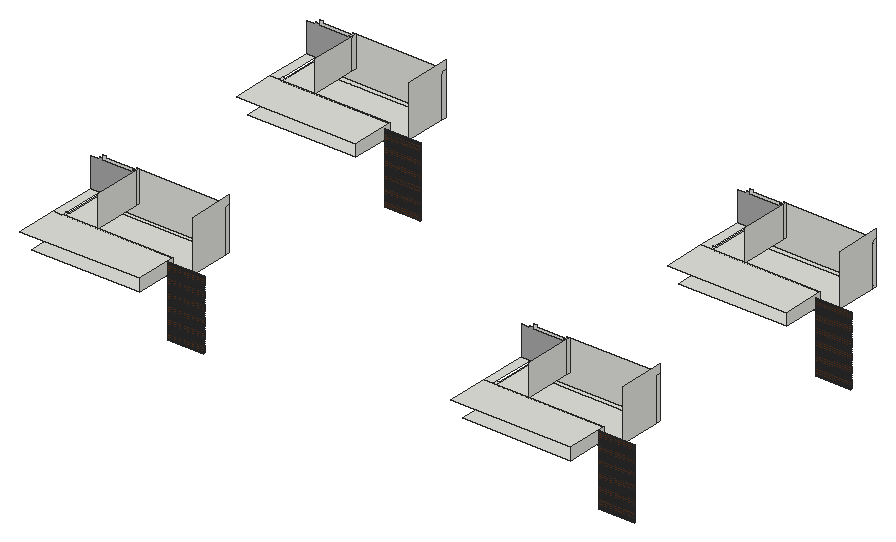
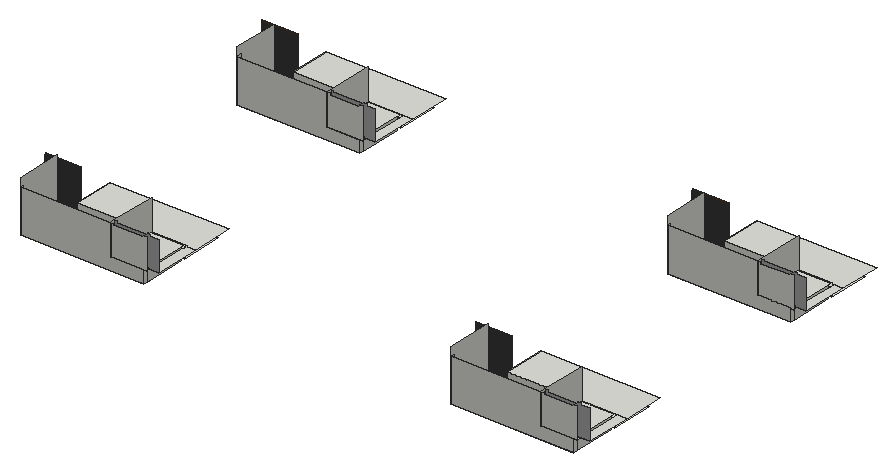
# SketchUp Ruby script. Lengths in inches.
U = 1.inch
M = Sketchup.active_model
def pt(a) = Geom::Point3d.new(a.map { |v| v * U })
def face(e, loops, mat)
  f = e.add_face(loops[0].map { |a| pt(a) })
  loops[1..].each { |l| e.add_face(l.map { |a| pt(a) }).erase! }
  f.material = f.back_material = mat if mat
  f
end
# faces: each face lists its corners as indices into pts; further lists are holes
def faces(e, pts, list, mat = nil) = list.each { |f| face(e, (f[0].is_a?(Array) ? f : [f]).map { |l| l.map { |i| pts[i] } }, mat) }
# xy, xz, yz: faces in a plane at the given z, y or x. An outline is a flat list of corners, or four numbers for a rectangle; further outlines are holes
def ring(l) = l.size == 4 ? [[l[0], l[1]], [l[2], l[1]], [l[2], l[3]], [l[0], l[3]]] : l.each_slice(2).to_a
def flat(e, list, mat, &to3) = list.each { |f| face(e, (f[0].is_a?(Array) ? f : [f]).map { |l| ring(l).map { |u, v| to3.(u, v) } }, mat) }
def xy(e, z, list, mat = nil) = flat(e, list, mat) { |x, y| [x, y, z] }
def xz(e, y, list, mat = nil) = flat(e, list, mat) { |x, z| [x, y, z] }
def yz(e, x, list, mat = nil) = flat(e, list, mat) { |y, z| [x, y, z] }
def lines(e, pts, list) = list.each { |a, b| e.add_line(pt(pts[a]), pt(pts[b])) }
# prism: a flat outline (further loops are holes) pulled along v
def prism(e, loops, v, mat = nil)
  f = face(e, loops, mat); d = Geom::Vector3d.new(v.map { |x| x * U })
  f.pushpull(f.normal.samedirection?(d) ? d.length : -d.length)
end
def box(e, o, s, mat = nil) = prism(e, [[o, [o[0] + s[0], o[1], o[2]], [o[0] + s[0], o[1] + s[1], o[2]], [o[0], o[1] + s[1], o[2]]]], [0, 0, s[2]], mat)
def at(x, y, z, deg = 0) = Geom::Transformation.translation(pt([x, y, z])) * Geom::Transformation.rotation(ORIGIN, Z_AXIS, deg.degrees)
def axes(o, x, y, z) = Geom::Transformation.new([*x, 0, *y, 0, *z, 0, *pt(o).to_a, 1])
def part(name) = M.definitions.add(name)
# library, detail: a bought-in or finely detailed component or shape, given as its bounding box
def library(name, o, s) = part(name).tap { |d| box(d.entities, o, s) }
def detail(e, o, s) = box(e.add_group.entities, o, s)
def put(e, d, t, mat = nil) = e.add_instance(d, t).tap { |i| i.material = mat if mat }
def group(e, t, mat = nil) = e.add_group.tap { |g| g.transformation = t; g.material = mat if mat }.entities
root = M.entities
M.materials.add("[Color M03]1").color = [170, 170, 170]
M.materials.add("[Wood Veneer 01]").color = [96, 56, 29]
c1 = library("A$C06767DEF\#1",[-8.3,1.21,0],[7.09,7.09,5.51])
xy(root,266.84,[[534.24,466.33,620.86,468.64],[1582.55,466.33,1669.17,468.64]])
xy(root,267.22,[[533.89,1125.42,620.51,1127.73],[1582.21,1125.42,1668.82,1127.73]])
xy(root,267.875,[[534.24,466.33,620.86,468.64],[1582.55,466.33,1669.17,468.64]])
xy(root,268.25,[[533.89,1125.42,620.51,1127.73],[1582.21,1125.42,1668.82,1127.73]])
xy(root,270.91,[[534.24,466.33,620.86,468.64],[1582.55,466.33,1669.17,468.64]])
xy(root,271.28,[[533.89,1125.42,620.51,1127.73],[1582.21,1125.42,1668.82,1127.73]])
xy(root,271.9375,[[534.24,466.33,620.86,468.64],[1582.55,466.33,1669.17,468.64]])
xy(root,272.3125,[[533.89,1125.42,620.51,1127.73],[1582.21,1125.42,1668.82,1127.73]])
xy(root,274.97,[[534.24,466.33,620.86,468.64],[1582.55,466.33,1669.17,468.64]])
xy(root,275.34,[[533.89,1125.42,620.51,1127.73],[1582.21,1125.42,1668.82,1127.73]])
xy(root,276,[[534.24,466.33,620.86,468.64],[1582.55,466.33,1669.17,468.64]])
xy(root,276.375,[[533.89,1125.42,620.51,1127.73],[1582.21,1125.42,1668.82,1127.73]])
xy(root,279.03,[[534.24,466.33,620.86,468.64],[1582.55,466.33,1669.17,468.64]])
xy(root,279.41,[[533.89,1125.42,620.51,1127.73],[1582.21,1125.42,1668.82,1127.73]])
xy(root,280.0625,[[534.24,466.33,620.86,468.64],[1582.55,466.33,1669.17,468.64]])
xy(root,280.4375,[[533.89,1125.42,620.51,1127.73],[1582.21,1125.42,1668.82,1127.73]])
xy(root,283.09,[[534.24,466.33,620.86,468.64],[1582.55,466.33,1669.17,468.64]])
xy(root,283.47,[[533.89,1125.42,620.51,1127.73],[1582.21,1125.42,1668.82,1127.73]])
xy(root,284.125,[[534.24,466.33,620.86,468.64],[1582.55,466.33,1669.17,468.64]])
xy(root,284.5,[[533.89,1125.42,620.51,1127.73],[1582.21,1125.42,1668.82,1127.73]])
xy(root,287.16,[[534.24,466.33,620.86,468.64],[1582.55,466.33,1669.17,468.64]])
xy(root,287.53,[[533.89,1125.42,620.51,1127.73],[1582.21,1125.42,1668.82,1127.73]])
xy(root,288.1875,[[534.24,466.33,620.86,468.64],[1582.55,466.33,1669.17,468.64]])
xy(root,288.5625,[[533.89,1125.42,620.51,1127.73],[1582.21,1125.42,1668.82,1127.73]])
xy(root,291.22,[[534.24,466.33,620.86,468.64],[1582.55,466.33,1669.17,468.64]])
xy(root,291.59,[[533.89,1125.42,620.51,1127.73],[1582.21,1125.42,1668.82,1127.73]])
xy(root,292.25,[[534.24,466.33,620.86,468.64],[1582.55,466.33,1669.17,468.64]])
xy(root,292.625,[[533.89,1125.42,620.51,1127.73],[1582.21,1125.42,1668.82,1127.73]])
xy(root,295.28,[[534.24,466.33,620.86,468.64],[1582.55,466.33,1669.17,468.64]])
xy(root,295.66,[[533.89,1125.42,620.51,1127.73],[1582.21,1125.42,1668.82,1127.73]])
xy(root,296.3125,[[534.24,466.33,620.86,468.64],[1582.55,466.33,1669.17,468.64]])
xy(root,296.6875,[[533.89,1125.42,620.51,1127.73],[1582.21,1125.42,1668.82,1127.73]])
xy(root,299.34,[[534.24,466.33,620.86,468.64],[1582.55,466.33,1669.17,468.64]])
xy(root,299.72,[[533.89,1125.42,620.51,1127.73],[1582.21,1125.42,1668.82,1127.73]])
xy(root,300.375,[[534.24,466.33,620.86,468.64],[1582.55,466.33,1669.17,468.64]])
xy(root,300.75,[[533.89,1125.42,620.51,1127.73],[1582.21,1125.42,1668.82,1127.73]])
xy(root,303.41,[[534.24,466.33,620.86,468.64],[1582.55,466.33,1669.17,468.64]])
xy(root,303.78,[[533.89,1125.42,620.51,1127.73],[1582.21,1125.42,1668.82,1127.73]])
xy(root,304.4375,[[534.24,466.33,620.86,468.64],[1582.55,466.33,1669.17,468.64]])
xy(root,304.8125,[[533.89,1125.42,620.51,1127.73],[1582.21,1125.42,1668.82,1127.73]])
xy(root,307.47,[[534.24,466.33,620.86,468.64],[1582.55,466.33,1669.17,468.64]])
xy(root,307.84,[[533.89,1125.42,620.51,1127.73],[1582.21,1125.42,1668.82,1127.73]])
xy(root,308.5,[[534.24,466.33,620.86,468.64],[1582.55,466.33,1669.17,468.64]])
xy(root,308.875,[[533.89,1125.42,620.51,1127.73],[1582.21,1125.42,1668.82,1127.73]])
xy(root,311.53,[[534.24,466.33,620.86,468.64],[1582.55,466.33,1669.17,468.64]])
xy(root,311.91,[[533.89,1125.42,620.51,1127.73],[1582.21,1125.42,1668.82,1127.73]])
xy(root,312.5625,[[534.24,466.33,620.86,468.64],[1582.55,466.33,1669.17,468.64]])
xy(root,312.9375,[[533.89,1125.42,620.51,1127.73],[1582.21,1125.42,1668.82,1127.73]])
xy(root,315.59,[[534.24,466.33,620.86,468.64],[1582.55,466.33,1669.17,468.64]])
xy(root,315.97,[[533.89,1125.42,620.51,1127.73],[1582.21,1125.42,1668.82,1127.73]])
xy(root,316.625,[[534.24,466.33,620.86,468.64],[1582.55,466.33,1669.17,468.64]])
xy(root,317,[[533.89,1125.42,620.51,1127.73],[1582.21,1125.42,1668.82,1127.73]])
xy(root,319.66,[[534.24,466.33,620.86,468.64],[1582.55,466.33,1669.17,468.64]])
xy(root,320.03,[[533.89,1125.42,620.51,1127.73],[1582.21,1125.42,1668.82,1127.73]])
xy(root,320.6875,[[534.24,466.33,620.86,468.64],[1582.55,466.33,1669.17,468.64]])
xy(root,321.0625,[[533.89,1125.42,620.51,1127.73],[1582.21,1125.42,1668.82,1127.73]])
xy(root,323.72,[[534.24,466.33,620.86,468.64],[1582.55,466.33,1669.17,468.64]])
xy(root,324.09,[[533.89,1125.42,620.51,1127.73],[1582.21,1125.42,1668.82,1127.73]])
xy(root,324.75,[[534.24,466.33,620.86,468.64],[1582.55,466.33,1669.17,468.64]])
xy(root,325.125,[[533.89,1125.42,620.51,1127.73],[1582.21,1125.42,1668.82,1127.73]])
xy(root,327.78,[[534.24,466.33,620.86,468.64],[1582.55,466.33,1669.17,468.64]])
xy(root,328.16,[[533.89,1125.42,620.51,1127.73],[1582.21,1125.42,1668.82,1127.73]])
xy(root,328.8125,[[534.24,466.33,620.86,468.64],[1582.55,466.33,1669.17,468.64]])
xy(root,329.1875,[[533.89,1125.42,620.51,1127.73],[1582.21,1125.42,1668.82,1127.73]])
xy(root,331.84,[[534.24,466.33,620.86,468.64],[1582.55,466.33,1669.17,468.64]])
xy(root,332.22,[[533.89,1125.42,620.51,1127.73],[1582.21,1125.42,1668.82,1127.73]])
xy(root,332.875,[[534.24,466.33,620.86,468.64],[1582.55,466.33,1669.17,468.64]])
xy(root,333.25,[[533.89,1125.42,620.51,1127.73],[1582.21,1125.42,1668.82,1127.73]])
xy(root,335.91,[[534.24,466.33,620.86,468.64],[1582.55,466.33,1669.17,468.64]])
xy(root,336.28,[[533.89,1125.42,620.51,1127.73],[1582.21,1125.42,1668.82,1127.73]])
xy(root,336.9375,[[534.24,466.33,620.86,468.64],[1582.55,466.33,1669.17,468.64]])
xy(root,337.3125,[[533.89,1125.42,620.51,1127.73],[1582.21,1125.42,1668.82,1127.73]])
xy(root,339.97,[[534.24,466.33,620.86,468.64],[1582.55,466.33,1669.17,468.64]])
xy(root,340.34,[[533.89,1125.42,620.51,1127.73],[1582.21,1125.42,1668.82,1127.73]])
xy(root,341,[[534.24,466.33,620.86,468.64],[1582.55,466.33,1669.17,468.64]])
xy(root,341.375,[[533.89,1125.42,620.51,1127.73],[1582.21,1125.42,1668.82,1127.73]])
xy(root,344.03,[[534.24,466.33,620.86,468.64],[1582.55,466.33,1669.17,468.64]])
xy(root,344.41,[[533.89,1125.42,620.51,1127.73],[1582.21,1125.42,1668.82,1127.73]])
xy(root,345.0625,[[534.24,466.33,620.86,468.64],[1582.55,466.33,1669.17,468.64]])
xy(root,345.4375,[[533.89,1125.42,620.51,1127.73],[1582.21,1125.42,1668.82,1127.73]])
xy(root,348.09,[[534.24,466.33,620.86,468.64],[1582.55,466.33,1669.17,468.64]])
xy(root,348.47,[[533.89,1125.42,620.51,1127.73],[1582.21,1125.42,1668.82,1127.73]])
xy(root,349.125,[[534.24,466.33,620.86,468.64],[1582.55,466.33,1669.17,468.64]])
xy(root,349.5,[[533.89,1125.42,620.51,1127.73],[1582.21,1125.42,1668.82,1127.73]])
xy(root,352.16,[[534.24,466.33,620.86,468.64],[1582.55,466.33,1669.17,468.64]])
xy(root,352.53,[[533.89,1125.42,620.51,1127.73],[1582.21,1125.42,1668.82,1127.73]])
xy(root,353.1875,[[534.24,466.33,620.86,468.64],[1582.55,466.33,1669.17,468.64]])
xy(root,353.5625,[[533.89,1125.42,620.51,1127.73],[1582.21,1125.42,1668.82,1127.73]])
xy(root,355.625,[[292.8,534.98,520.24,546.92],[1341.11,534.98,1568.55,546.92]])
xy(root,356.22,[[534.24,466.33,620.86,468.64],[1582.55,466.33,1669.17,468.64]])
xy(root,356.59,[[533.89,1125.42,620.51,1127.73],[1582.21,1125.42,1668.82,1127.73]])
xy(root,357.25,[[534.24,466.33,620.86,468.64],[1582.55,466.33,1669.17,468.64]])
xy(root,357.625,[[533.89,1125.42,620.51,1127.73],[1582.21,1125.42,1668.82,1127.73]])
xy(root,360.0625,[[292.46,1194.07,519.89,1206.01],[1340.77,1194.07,1568.21,1206.01]])
xy(root,360.28,[[534.24,466.33,620.86,468.64],[1582.55,466.33,1669.17,468.64]])
xy(root,360.66,[[533.89,1125.42,620.51,1127.73],[1582.21,1125.42,1668.82,1127.73]])
xy(root,361.3125,[[534.24,466.33,620.86,468.64],[1582.55,466.33,1669.17,468.64]])
xy(root,361.6875,[[533.89,1125.42,620.51,1127.73],[1582.21,1125.42,1668.82,1127.73]])
xy(root,364.34,[[534.24,466.33,620.86,468.64],[1582.55,466.33,1669.17,468.64]])
xy(root,364.72,[[533.89,1125.42,620.51,1127.73],[1582.21,1125.42,1668.82,1127.73]])
xy(root,365.375,[[534.24,466.33,620.86,468.64],[1582.55,466.33,1669.17,468.64]])
xy(root,365.75,[[533.89,1125.42,620.51,1127.73],[1582.21,1125.42,1668.82,1127.73]])
xy(root,368.41,[[534.24,466.33,620.86,468.64],[1582.55,466.33,1669.17,468.64]])
xy(root,368.78,[[533.89,1125.42,620.51,1127.73],[1582.21,1125.42,1668.82,1127.73]])
xy(root,369.4375,[[534.24,466.33,620.86,468.64],[1582.55,466.33,1669.17,468.64]])
xy(root,369.8125,[[533.89,1125.42,620.51,1127.73],[1582.21,1125.42,1668.82,1127.73]])
xy(root,370.64,[[228.06,433.78,490.99,534.98],[1276.37,433.78,1539.31,534.98],[228.06,546.92,528.37,647.98],[1276.37,546.92,1576.68,647.98],[228.06,647.98,528.37,659.09],
  [1276.37,647.98,1576.68,659.09]])
xy(root,372.47,[[534.24,466.33,620.86,468.64],[1582.55,466.33,1669.17,468.64]])
xy(root,372.84,[[533.89,1125.42,620.51,1127.73],[1582.21,1125.42,1668.82,1127.73]])
xy(root,373.5,[[534.24,466.33,620.86,468.64],[1582.55,466.33,1669.17,468.64]])
xy(root,373.875,[[533.89,1125.42,620.51,1127.73],[1582.21,1125.42,1668.82,1127.73]])
xy(root,375.08,[[227.71,1092.87,490.65,1194.07],[1276.02,1092.87,1538.96,1194.07],[227.71,1206.01,528.02,1307.07],[1276.02,1206.01,1576.34,1307.07],[227.71,1307.07,528.02,1318.18],
  [1276.02,1307.07,1576.34,1318.18]])
xy(root,376.53,[[534.24,466.33,620.86,468.64],[1582.55,466.33,1669.17,468.64]])
xy(root,376.91,[[533.89,1125.42,620.51,1127.73],[1582.21,1125.42,1668.82,1127.73]])
xy(root,377.5625,[[534.24,466.33,620.86,468.64],[1582.55,466.33,1669.17,468.64]])
xy(root,377.9375,[[533.89,1125.42,620.51,1127.73],[1582.21,1125.42,1668.82,1127.73]])
xy(root,380.59,[[534.24,466.33,620.86,468.64],[1582.55,466.33,1669.17,468.64]])
xy(root,380.97,[[533.89,1125.42,620.51,1127.73],[1582.21,1125.42,1668.82,1127.73]])
xy(root,381.625,[[534.24,466.33,620.86,468.64],[1582.55,466.33,1669.17,468.64]])
xy(root,382,[[533.89,1125.42,620.51,1127.73],[1582.21,1125.42,1668.82,1127.73]])
xy(root,384.66,[[534.24,466.33,620.86,468.64],[1582.55,466.33,1669.17,468.64]])
xy(root,385.03,[[533.89,1125.42,620.51,1127.73],[1582.21,1125.42,1668.82,1127.73]])
xy(root,385.6875,[[534.24,466.33,620.86,468.64],[1582.55,466.33,1669.17,468.64]])
xy(root,386.0625,[[533.89,1125.42,620.51,1127.73],[1582.21,1125.42,1668.82,1127.73]])
xy(root,388.72,[[534.24,466.33,620.86,468.64],[1582.55,466.33,1669.17,468.64]])
xy(root,389.09,[[533.89,1125.42,620.51,1127.73],[1582.21,1125.42,1668.82,1127.73]])
xy(root,389.75,[[534.24,466.33,620.86,468.64],[1582.55,466.33,1669.17,468.64]])
xy(root,390.125,[[533.89,1125.42,620.51,1127.73],[1582.21,1125.42,1668.82,1127.73]])
xy(root,392.78,[[534.24,466.33,620.86,468.64],[1582.55,466.33,1669.17,468.64]])
xy(root,393.16,[[533.89,1125.42,620.51,1127.73],[1582.21,1125.42,1668.82,1127.73]])
xy(root,393.8125,[[534.24,466.33,620.86,468.64],[1582.55,466.33,1669.17,468.64]])
xy(root,394.1875,[[533.89,1125.42,620.51,1127.73],[1582.21,1125.42,1668.82,1127.73]])
xy(root,396.84,[[534.24,466.33,620.86,468.64],[1582.55,466.33,1669.17,468.64]])
xy(root,397.22,[[533.89,1125.42,620.51,1127.73],[1582.21,1125.42,1668.82,1127.73]])
xy(root,397.875,[[534.24,466.33,620.86,468.64],[1582.55,466.33,1669.17,468.64]])
xy(root,398.25,[[533.89,1125.42,620.51,1127.73],[1582.21,1125.42,1668.82,1127.73]])
xy(root,400,[[200.03,433.78,490.99,534.98],[1248.34,433.78,1539.31,534.98],[200.03,534.98,221.15,647.98],[221.15,534.98,228.06,546.92],[228.06,534.98,308.65,647.98],
  [1248.34,534.98,1269.46,647.98],[1269.46,534.98,1276.37,546.92],[1276.37,534.98,1356.97,647.98],[221.15,647.98,228.06,659.09],[228.06,647.98,308.65,659.09],
  [1269.46,647.98,1276.37,659.09],[1276.37,647.98,1356.97,659.09]])
xy(root,400.91,[[534.24,466.33,620.86,468.64],[1582.55,466.33,1669.17,468.64]])
xy(root,401.28,[[533.89,1125.42,620.51,1127.73],[1582.21,1125.42,1668.82,1127.73]])
xy(root,401.9375,[[534.24,466.33,620.86,468.64],[1582.55,466.33,1669.17,468.64]])
xy(root,402.3125,[[533.89,1125.42,620.51,1127.73],[1582.21,1125.42,1668.82,1127.73]])
xy(root,404.4375,[[199.6875,1092.87,490.65,1194.07],[1248,1092.87,1538.96,1194.07],[199.6875,1194.07,220.81,1307.07],[220.81,1194.07,227.71,1206.01],[227.71,1194.07,308.31,1307.07],
  [1248,1194.07,1269.12,1307.07],[1269.12,1194.07,1276.02,1206.01],[1276.02,1194.07,1356.62,1307.07],[220.81,1307.07,227.71,1318.18],[227.71,1307.07,308.31,1318.18],
  [1269.12,1307.07,1276.02,1318.18],[1276.02,1307.07,1356.62,1318.18]])
xy(root,404.97,[[534.24,466.33,620.86,468.64],[1582.55,466.33,1669.17,468.64]])
xy(root,405.34,[[533.89,1125.42,620.51,1127.73],[1582.21,1125.42,1668.82,1127.73]])
xy(root,406,[[534.24,466.33,620.86,468.64],[1582.55,466.33,1669.17,468.64]])
xy(root,406.375,[[533.89,1125.42,620.51,1127.73],[1582.21,1125.42,1668.82,1127.73]])
xy(root,409.03,[[534.24,466.33,620.86,468.64],[1582.55,466.33,1669.17,468.64]])
xy(root,409.41,[[533.89,1125.42,620.51,1127.73],[1582.21,1125.42,1668.82,1127.73]])
xy(root,410.0625,[[534.24,466.33,620.86,468.64],[1582.55,466.33,1669.17,468.64]])
xy(root,410.4375,[[533.89,1125.42,620.51,1127.73],[1582.21,1125.42,1668.82,1127.73]])
xy(root,413.09,[[534.24,466.33,620.86,468.64],[1582.55,466.33,1669.17,468.64]])
xy(root,413.47,[[533.89,1125.42,620.51,1127.73],[1582.21,1125.42,1668.82,1127.73]])
xy(root,414.125,[[534.24,466.33,620.86,468.64],[1582.55,466.33,1669.17,468.64]])
xy(root,414.5,[[533.89,1125.42,620.51,1127.73],[1582.21,1125.42,1668.82,1127.73]])
xy(root,417.16,[[534.24,466.33,620.86,468.64],[1582.55,466.33,1669.17,468.64]])
xy(root,417.53,[[533.89,1125.42,620.51,1127.73],[1582.21,1125.42,1668.82,1127.73]])
xy(root,418.1875,[[534.24,466.33,620.86,468.64],[1582.55,466.33,1669.17,468.64]])
xy(root,418.5625,[[533.89,1125.42,620.51,1127.73],[1582.21,1125.42,1668.82,1127.73]])
xy(root,421.22,[[534.24,466.33,620.86,468.64],[1582.55,466.33,1669.17,468.64]])
xy(root,421.59,[[533.89,1125.42,620.51,1127.73],[1582.21,1125.42,1668.82,1127.73]])
xy(root,422.25,[[534.24,466.33,620.86,468.64],[1582.55,466.33,1669.17,468.64]])
xy(root,422.625,[[533.89,1125.42,620.51,1127.73],[1582.21,1125.42,1668.82,1127.73]])
xy(root,425.28,[[534.24,466.33,620.86,468.64],[1582.55,466.33,1669.17,468.64]])
xy(root,425.66,[[533.89,1125.42,620.51,1127.73],[1582.21,1125.42,1668.82,1127.73]])
xy(root,426.3125,[[534.24,466.33,620.86,468.64],[1582.55,466.33,1669.17,468.64]])
xy(root,426.6875,[[533.89,1125.42,620.51,1127.73],[1582.21,1125.42,1668.82,1127.73]])
xy(root,429.34,[[534.24,466.33,620.86,468.64],[1582.55,466.33,1669.17,468.64]])
xy(root,429.72,[[533.89,1125.42,620.51,1127.73],[1582.21,1125.42,1668.82,1127.73]])
xy(root,430.375,[[534.24,466.33,620.86,468.64],[1582.55,466.33,1669.17,468.64]])
xy(root,430.75,[[533.89,1125.42,620.51,1127.73],[1582.21,1125.42,1668.82,1127.73]])
xy(root,433.41,[[534.24,466.33,620.86,468.64],[1582.55,466.33,1669.17,468.64]])
xy(root,433.78,[[533.89,1125.42,620.51,1127.73],[1582.21,1125.42,1668.82,1127.73]])
xy(root,434.4375,[[534.24,466.33,620.86,468.64],[1582.55,466.33,1669.17,468.64]])
xy(root,434.8125,[[533.89,1125.42,620.51,1127.73],[1582.21,1125.42,1668.82,1127.73]])
xz(root,466.33,[[534.24,267.875,620.86,270.91],[1582.55,267.875,1669.17,270.91],[534.24,271.9375,620.86,274.97],[1582.55,271.9375,1669.17,274.97],[534.24,276,620.86,279.03],
  [1582.55,276,1669.17,279.03],[534.24,280.0625,620.86,283.09],[1582.55,280.0625,1669.17,283.09],[534.24,284.125,620.86,287.16],[1582.55,284.125,1669.17,287.16],
  [534.24,288.1875,620.86,291.22],[1582.55,288.1875,1669.17,291.22],[534.24,292.25,620.86,295.28],[1582.55,292.25,1669.17,295.28],[534.24,296.3125,620.86,299.34],
  [1582.55,296.3125,1669.17,299.34],[534.24,300.375,620.86,303.41],[1582.55,300.375,1669.17,303.41],[534.24,304.4375,620.86,307.47],[1582.55,304.4375,1669.17,307.47],
  [534.24,308.5,620.86,311.53],[1582.55,308.5,1669.17,311.53],[534.24,312.5625,620.86,315.59],[1582.55,312.5625,1669.17,315.59],[534.24,316.625,620.86,319.66],
  [1582.55,316.625,1669.17,319.66],[534.24,320.6875,620.86,323.72],[1582.55,320.6875,1669.17,323.72],[534.24,324.75,620.86,327.78],[1582.55,324.75,1669.17,327.78],
  [534.24,328.8125,620.86,331.84],[1582.55,328.8125,1669.17,331.84],[534.24,332.875,620.86,335.91],[1582.55,332.875,1669.17,335.91],[534.24,336.9375,620.86,339.97],
  [1582.55,336.9375,1669.17,339.97],[534.24,341,620.86,344.03],[1582.55,341,1669.17,344.03],[534.24,345.0625,620.86,348.09],[1582.55,345.0625,1669.17,348.09],
  [534.24,349.125,620.86,352.16],[1582.55,349.125,1669.17,352.16],[534.24,353.1875,620.86,356.22],[1582.55,353.1875,1669.17,356.22],[534.24,357.25,620.86,360.28],
  [1582.55,357.25,1669.17,360.28],[534.24,361.3125,620.86,364.34],[1582.55,361.3125,1669.17,364.34],[534.24,365.375,620.86,368.41],[1582.55,365.375,1669.17,368.41],
  [534.24,369.4375,620.86,372.47],[1582.55,369.4375,1669.17,372.47],[534.24,373.5,620.86,376.53],[1582.55,373.5,1669.17,376.53],[534.24,377.5625,620.86,380.59],
  [1582.55,377.5625,1669.17,380.59],[534.24,381.625,620.86,384.66],[1582.55,381.625,1669.17,384.66],[534.24,385.6875,620.86,388.72],[1582.55,385.6875,1669.17,388.72],
  [534.24,389.75,620.86,392.78],[1582.55,389.75,1669.17,392.78],[534.24,393.8125,620.86,396.84],[1582.55,393.8125,1669.17,396.84],[534.24,397.875,620.86,400.91],
  [1582.55,397.875,1669.17,400.91],[534.24,401.9375,620.86,404.97],[1582.55,401.9375,1669.17,404.97],[534.24,406,620.86,409.03],[1582.55,406,1669.17,409.03],
  [534.24,410.0625,620.86,413.09],[1582.55,410.0625,1669.17,413.09],[534.24,414.125,620.86,417.16],[1582.55,414.125,1669.17,417.16],[534.24,418.1875,620.86,421.22],
  [1582.55,418.1875,1669.17,421.22],[534.24,422.25,620.86,425.28],[1582.55,422.25,1669.17,425.28],[534.24,426.3125,620.86,429.34],[1582.55,426.3125,1669.17,429.34],
  [534.24,430.375,620.86,433.41],[1582.55,430.375,1669.17,433.41],[534.24,434.4375,620.86,437.47],[1582.55,434.4375,1669.17,437.47]],"[Wood Veneer 01]")
xz(root,468.64,[[534.24,266.84,620.86,267.875],[1582.55,266.84,1669.17,267.875],[534.24,270.91,620.86,271.9375],[1582.55,270.91,1669.17,271.9375],[534.24,274.97,620.86,276],
  [1582.55,274.97,1669.17,276],[534.24,279.03,620.86,280.0625],[1582.55,279.03,1669.17,280.0625],[534.24,283.09,620.86,284.125],[1582.55,283.09,1669.17,284.125],
  [534.24,291.22,620.86,292.25],[1582.55,291.22,1669.17,292.25],[534.24,295.28,620.86,296.3125],[1582.55,295.28,1669.17,296.3125],[534.24,299.34,620.86,300.375],
  [1582.55,299.34,1669.17,300.375],[534.24,303.41,620.86,304.4375],[1582.55,303.41,1669.17,304.4375],[534.24,307.47,620.86,308.5],[1582.55,307.47,1669.17,308.5],
  [534.24,311.53,620.86,312.5625],[1582.55,311.53,1669.17,312.5625],[534.24,315.59,620.86,316.625],[1582.55,315.59,1669.17,316.625],[534.24,319.66,620.86,320.6875],
  [1582.55,319.66,1669.17,320.6875],[534.24,323.72,620.86,324.75],[1582.55,323.72,1669.17,324.75],[534.24,327.78,620.86,328.8125],[1582.55,327.78,1669.17,328.8125],
  [534.24,331.84,620.86,332.875],[1582.55,331.84,1669.17,332.875],[534.24,335.91,620.86,336.9375],[1582.55,335.91,1669.17,336.9375],[534.24,339.97,620.86,341],
  [1582.55,339.97,1669.17,341],[534.24,344.03,620.86,345.0625],[1582.55,344.03,1669.17,345.0625],[534.24,348.09,620.86,349.125],[1582.55,348.09,1669.17,349.125],
  [534.24,352.16,620.86,353.1875],[1582.55,352.16,1669.17,353.1875],[534.24,356.22,620.86,357.25],[1582.55,356.22,1669.17,357.25],[534.24,360.28,620.86,361.3125],
  [1582.55,360.28,1669.17,361.3125],[534.24,364.34,620.86,365.375],[1582.55,364.34,1669.17,365.375],[534.24,368.41,620.86,369.4375],[1582.55,368.41,1669.17,369.4375],
  [534.24,372.47,620.86,373.5],[1582.55,372.47,1669.17,373.5],[534.24,376.53,620.86,377.5625],[1582.55,376.53,1669.17,377.5625],[534.24,380.59,620.86,381.625],
  [1582.55,380.59,1669.17,381.625],[534.24,384.66,620.86,385.6875],[1582.55,384.66,1669.17,385.6875],[534.24,388.72,620.86,389.75],[1582.55,388.72,1669.17,389.75],
  [534.24,392.78,620.86,393.8125],[1582.55,392.78,1669.17,393.8125],[534.24,396.84,620.86,397.875],[1582.55,396.84,1669.17,397.875],[534.24,400.91,620.86,401.9375],
  [1582.55,400.91,1669.17,401.9375],[534.24,404.97,620.86,406],[1582.55,404.97,1669.17,406],[534.24,409.03,620.86,410.0625],[1582.55,409.03,1669.17,410.0625],
  [534.24,413.09,620.86,414.125],[1582.55,413.09,1669.17,414.125],[534.24,417.16,620.86,418.1875],[1582.55,417.16,1669.17,418.1875],[534.24,421.22,620.86,422.25],
  [1582.55,421.22,1669.17,422.25],[534.24,425.28,620.86,426.3125],[1582.55,425.28,1669.17,426.3125],[534.24,429.34,620.86,430.375],[1582.55,429.34,1669.17,430.375],
  [534.24,433.41,620.86,434.4375],[1582.55,433.41,1669.17,434.4375]])
xz(root,468.64,[[534.24,287.16,620.86,288.1875],[1582.55,287.16,1669.17,288.1875]],"[Wood Veneer 01]")
xz(root,534.98,[[228.06,370.64,490.99,400],[1276.37,370.64,1539.31,400]])
xz(root,647.98,[[200.03,400,308.65,400,308.65,475.57,302.29,475.57,302.29,471.94,228.06,471.94,228.06,475.57,221.15,475.57,221.15,471.94,200.03,471.94],[1248.34,400,1356.97,400,1356.97,475.57,1350.61,475.57,1350.61,471.94,1276.37,471.94,1276.37,475.57,1269.46,475.57,1269.46,471.94,1248.34,471.94]],"[Color M03]1")
xz(root,659.09,[[228.06,370.64,228.06,400,308.65,400,308.65,475.57,528.37,475.57,528.37,370.64],[1276.37,370.64,1276.37,400,1356.97,400,1356.97,475.57,1576.68,475.57,1576.68,370.64],[221.15,400,221.15,475.57,228.06,475.57,228.06,471.94,302.29,471.94,302.29,475.57,308.65,475.57,308.65,400],[1269.46,400,1269.46,475.57,1276.37,475.57,1276.37,471.94,1350.61,471.94,1350.61,475.57,1356.97,475.57,1356.97,400]])
xz(root,1125.42,[[533.89,268.25,620.51,271.28],[1582.21,268.25,1668.82,271.28],[533.89,272.3125,620.51,275.34],[1582.21,272.3125,1668.82,275.34],[533.89,276.375,620.51,279.41],
  [1582.21,276.375,1668.82,279.41],[533.89,280.4375,620.51,283.47],[1582.21,280.4375,1668.82,283.47],[533.89,284.5,620.51,287.53],[1582.21,284.5,1668.82,287.53],
  [533.89,288.5625,620.51,291.59],[1582.21,288.5625,1668.82,291.59],[533.89,292.625,620.51,295.66],[1582.21,292.625,1668.82,295.66],[533.89,296.6875,620.51,299.72],
  [1582.21,296.6875,1668.82,299.72],[533.89,300.75,620.51,303.78],[1582.21,300.75,1668.82,303.78],[533.89,304.8125,620.51,307.84],[1582.21,304.8125,1668.82,307.84],
  [533.89,308.875,620.51,311.91],[1582.21,308.875,1668.82,311.91],[533.89,312.9375,620.51,315.97],[1582.21,312.9375,1668.82,315.97],[533.89,317,620.51,320.03],
  [1582.21,317,1668.82,320.03],[533.89,321.0625,620.51,324.09],[1582.21,321.0625,1668.82,324.09],[533.89,325.125,620.51,328.16],[1582.21,325.125,1668.82,328.16],
  [533.89,329.1875,620.51,332.22],[1582.21,329.1875,1668.82,332.22],[533.89,333.25,620.51,336.28],[1582.21,333.25,1668.82,336.28],[533.89,337.3125,620.51,340.34],
  [1582.21,337.3125,1668.82,340.34],[533.89,341.375,620.51,344.41],[1582.21,341.375,1668.82,344.41],[533.89,345.4375,620.51,348.47],[1582.21,345.4375,1668.82,348.47],
  [533.89,349.5,620.51,352.53],[1582.21,349.5,1668.82,352.53],[533.89,353.5625,620.51,356.59],[1582.21,353.5625,1668.82,356.59],[533.89,357.625,620.51,360.66],
  [1582.21,357.625,1668.82,360.66],[533.89,361.6875,620.51,364.72],[1582.21,361.6875,1668.82,364.72],[533.89,365.75,620.51,368.78],[1582.21,365.75,1668.82,368.78],
  [533.89,369.8125,620.51,372.84],[1582.21,369.8125,1668.82,372.84],[533.89,373.875,620.51,376.91],[1582.21,373.875,1668.82,376.91],[533.89,377.9375,620.51,380.97],
  [1582.21,377.9375,1668.82,380.97],[533.89,382,620.51,385.03],[1582.21,382,1668.82,385.03],[533.89,386.0625,620.51,389.09],[1582.21,386.0625,1668.82,389.09],
  [533.89,390.125,620.51,393.16],[1582.21,390.125,1668.82,393.16],[533.89,394.1875,620.51,397.22],[1582.21,394.1875,1668.82,397.22],[533.89,398.25,620.51,401.28],
  [1582.21,398.25,1668.82,401.28],[533.89,402.3125,620.51,405.34],[1582.21,402.3125,1668.82,405.34],[533.89,406.375,620.51,409.41],[1582.21,406.375,1668.82,409.41],
  [533.89,410.4375,620.51,413.47],[1582.21,410.4375,1668.82,413.47],[533.89,414.5,620.51,417.53],[1582.21,414.5,1668.82,417.53],[533.89,418.5625,620.51,421.59],
  [1582.21,418.5625,1668.82,421.59],[533.89,422.625,620.51,425.66],[1582.21,422.625,1668.82,425.66],[533.89,426.6875,620.51,429.72],[1582.21,426.6875,1668.82,429.72],
  [533.89,430.75,620.51,433.78],[1582.21,430.75,1668.82,433.78],[533.89,434.8125,620.51,437.84],[1582.21,434.8125,1668.82,437.84]],"[Wood Veneer 01]")
xz(root,1127.73,[[533.89,267.22,620.51,268.25],[1582.21,267.22,1668.82,268.25],[533.89,271.28,620.51,272.3125],[1582.21,271.28,1668.82,272.3125],[533.89,275.34,620.51,276.375],
  [1582.21,275.34,1668.82,276.375],[533.89,279.41,620.51,280.4375],[1582.21,279.41,1668.82,280.4375],[533.89,283.47,620.51,284.5],[1582.21,283.47,1668.82,284.5],
  [533.89,287.53,620.51,288.5625],[1582.21,287.53,1668.82,288.5625],[533.89,295.66,620.51,296.6875],[1582.21,295.66,1668.82,296.6875],[533.89,299.72,620.51,300.75],
  [1582.21,299.72,1668.82,300.75],[533.89,303.78,620.51,304.8125],[1582.21,303.78,1668.82,304.8125],[533.89,307.84,620.51,308.875],[1582.21,307.84,1668.82,308.875],
  [533.89,311.91,620.51,312.9375],[1582.21,311.91,1668.82,312.9375],[533.89,315.97,620.51,317],[1582.21,315.97,1668.82,317],[533.89,320.03,620.51,321.0625],
  [1582.21,320.03,1668.82,321.0625],[533.89,324.09,620.51,325.125],[1582.21,324.09,1668.82,325.125],[533.89,328.16,620.51,329.1875],[1582.21,328.16,1668.82,329.1875],
  [533.89,332.22,620.51,333.25],[1582.21,332.22,1668.82,333.25],[533.89,336.28,620.51,337.3125],[1582.21,336.28,1668.82,337.3125],[533.89,340.34,620.51,341.375],
  [1582.21,340.34,1668.82,341.375],[533.89,344.41,620.51,345.4375],[1582.21,344.41,1668.82,345.4375],[533.89,348.47,620.51,349.5],[1582.21,348.47,1668.82,349.5],
  [533.89,352.53,620.51,353.5625],[1582.21,352.53,1668.82,353.5625],[533.89,356.59,620.51,357.625],[1582.21,356.59,1668.82,357.625],[533.89,360.66,620.51,361.6875],
  [1582.21,360.66,1668.82,361.6875],[533.89,364.72,620.51,365.75],[1582.21,364.72,1668.82,365.75],[533.89,368.78,620.51,369.8125],[1582.21,368.78,1668.82,369.8125],
  [533.89,372.84,620.51,373.875],[1582.21,372.84,1668.82,373.875],[533.89,376.91,620.51,377.9375],[1582.21,376.91,1668.82,377.9375],[533.89,380.97,620.51,382],
  [1582.21,380.97,1668.82,382],[533.89,385.03,620.51,386.0625],[1582.21,385.03,1668.82,386.0625],[533.89,389.09,620.51,390.125],[1582.21,389.09,1668.82,390.125],
  [533.89,393.16,620.51,394.1875],[1582.21,393.16,1668.82,394.1875],[533.89,397.22,620.51,398.25],[1582.21,397.22,1668.82,398.25],[533.89,401.28,620.51,402.3125],
  [1582.21,401.28,1668.82,402.3125],[533.89,405.34,620.51,406.375],[1582.21,405.34,1668.82,406.375],[533.89,409.41,620.51,410.4375],[1582.21,409.41,1668.82,410.4375],
  [533.89,413.47,620.51,414.5],[1582.21,413.47,1668.82,414.5],[533.89,417.53,620.51,418.5625],[1582.21,417.53,1668.82,418.5625],[533.89,421.59,620.51,422.625],
  [1582.21,421.59,1668.82,422.625],[533.89,425.66,620.51,426.6875],[1582.21,425.66,1668.82,426.6875],[533.89,429.72,620.51,430.75],[1582.21,429.72,1668.82,430.75],
  [533.89,433.78,620.51,434.8125],[1582.21,433.78,1668.82,434.8125]])
xz(root,1127.73,[[533.89,291.59,620.51,292.625],[1582.21,291.59,1668.82,292.625]],"[Wood Veneer 01]")
xz(root,1194.07,[[227.71,375.08,490.65,404.4375],[1276.02,375.08,1538.96,404.4375]])
xz(root,1307.07,[[199.6875,404.4375,308.31,404.4375,308.31,480,301.95,480,301.95,476.38,227.71,476.38,227.71,480,220.81,480,220.81,476.38,199.6875,476.38],[1248,404.4375,1356.62,404.4375,1356.62,480,1350.26,480,1350.26,476.38,1276.02,476.38,1276.02,480,1269.12,480,1269.12,476.38,1248,476.38]],"[Color M03]1")
xz(root,1318.18,[[227.71,375.08,227.71,404.4375,308.31,404.4375,308.31,480,528.02,480,528.02,375.08],[1276.02,375.08,1276.02,404.4375,1356.62,404.4375,1356.62,480,1576.34,480,1576.34,375.08],[220.81,404.4375,220.81,480,227.71,480,227.71,476.38,301.95,476.38,301.95,480,308.31,480,308.31,404.4375],[1269.12,404.4375,1269.12,480,1276.02,480,1276.02,476.38,1350.26,476.38,1350.26,480,1356.62,480,1356.62,404.4375]])
yz(root,227.71,[[1206.01,375.08,1307.07,404.4375],[1307.07,375.08,1318.18,404.4375]])
yz(root,228.06,[[546.92,370.64,647.98,400],[647.98,370.64,659.09,400]])
yz(root,308.31,[[1194.07,404.4375,1307.07,480],[1307.07,404.4375,1318.18,480]])
yz(root,308.65,[[534.98,400,647.98,475.57],[647.98,400,659.09,475.57]])
yz(root,490.65,[[1092.87,375.08,1194.07,404.4375]])
yz(root,490.99,[[433.78,370.64,534.98,400]])
yz(root,528.02,[[1206.01,375.08,1307.07,375.08,1307.07,480,1318.18,480,1318.18,500.5,1206.01,500.5],[1307.07,375.08,1318.18,480]])
yz(root,528.37,[[546.92,370.64,647.98,370.64,647.98,475.57,659.09,475.57,659.09,496.07,546.92,496.07],[647.98,370.64,659.09,475.57]])
yz(root,1276.02,[[1206.01,375.08,1307.07,404.4375],[1307.07,375.08,1318.18,404.4375]])
yz(root,1276.37,[[546.92,370.64,647.98,400],[647.98,370.64,659.09,400]])
yz(root,1356.62,[[1194.07,404.4375,1307.07,480],[1307.07,404.4375,1318.18,480]])
yz(root,1356.97,[[534.98,400,647.98,475.57],[647.98,400,659.09,475.57]])
yz(root,1538.96,[[1092.87,375.08,1194.07,404.4375]])
yz(root,1539.31,[[433.78,370.64,534.98,400]])
yz(root,1576.34,[[1206.01,375.08,1307.07,375.08,1307.07,480,1318.18,480,1318.18,500.5,1206.01,500.5],[1307.07,375.08,1318.18,480]])
yz(root,1576.68,[[546.92,370.64,647.98,370.64,647.98,475.57,659.09,475.57,659.09,496.07,546.92,496.07],[647.98,370.64,659.09,475.57]])
p = [[528.37,534.98,370.64],[528.37,546.92,370.64],[1576.68,534.98,370.64],[1576.68,546.92,370.64],[528.02,1194.07,375.08],[528.02,1206.01,375.08],
  [1576.34,1194.07,375.08],[1576.34,1206.01,375.08]]
lines(root,p,[[0,1],[2,3],[4,5],[6,7]])
put(root,c1,at(249.3,477.92,365.125))
put(root,c1,at(313.92,477.92,365.125))
put(root,c1,at(371.11,477.92,365.125))
put(root,c1,at(446.48,477.92,365.125))
put(root,c1,at(1297.61,477.92,365.125))
put(root,c1,at(1362.23,477.92,365.125))
put(root,c1,at(1494.8,477.92,365.125))
put(root,c1,at(1419.42,477.92,365.125))
put(root,c1,at(248.95,1137.01,369.5625))
put(root,c1,at(313.58,1137.01,369.5625))
put(root,c1,at(446.14,1137.01,369.5625))
put(root,c1,at(370.77,1137.01,369.5625))
put(root,c1,at(1494.45,1137.01,369.5625))
put(root,c1,at(1419.08,1137.01,369.5625))
put(root,c1,at(1297.27,1137.01,369.5625))
put(root,c1,at(1361.89,1137.01,369.5625))
